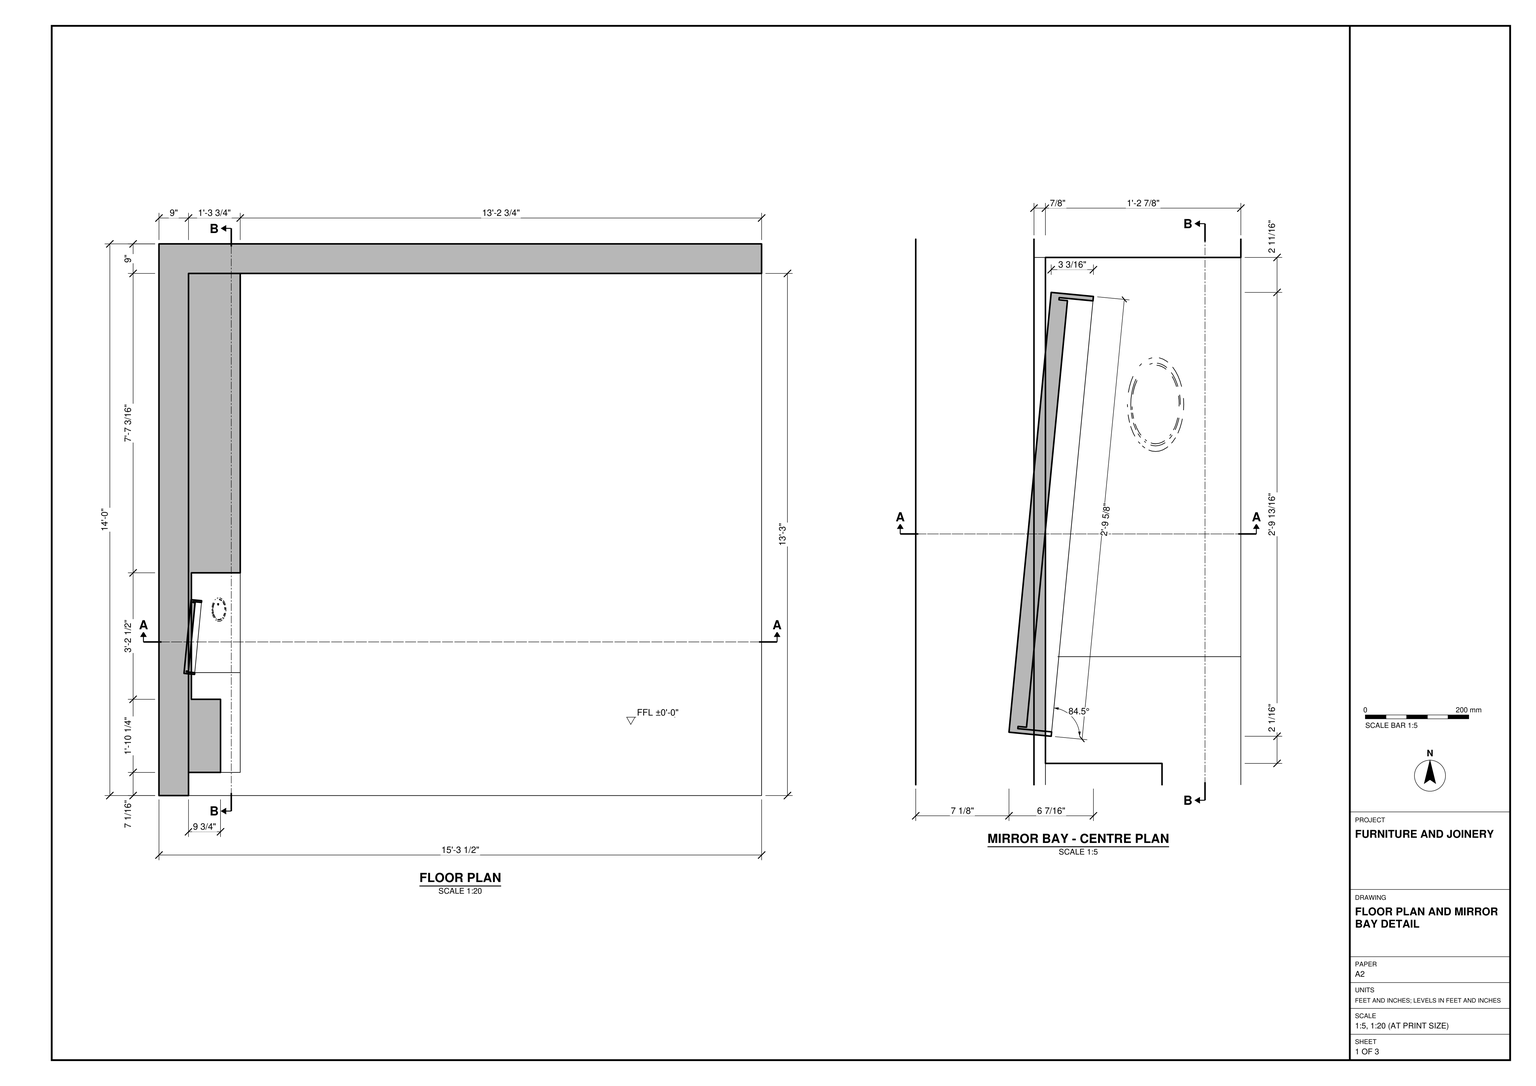
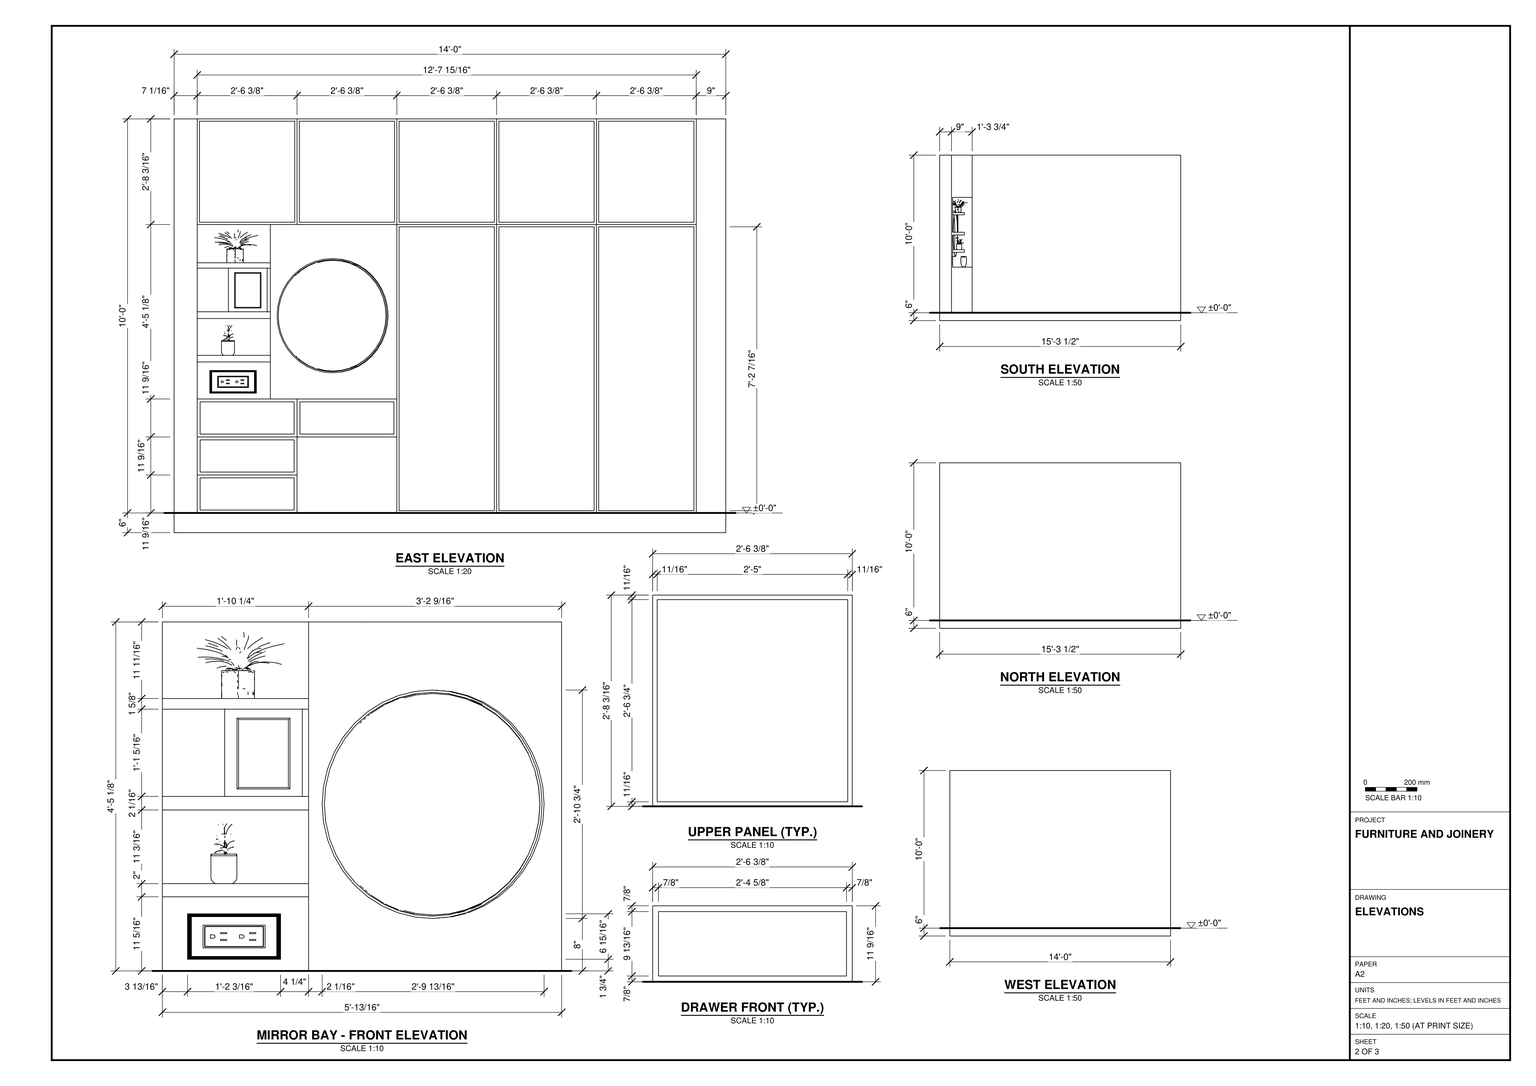
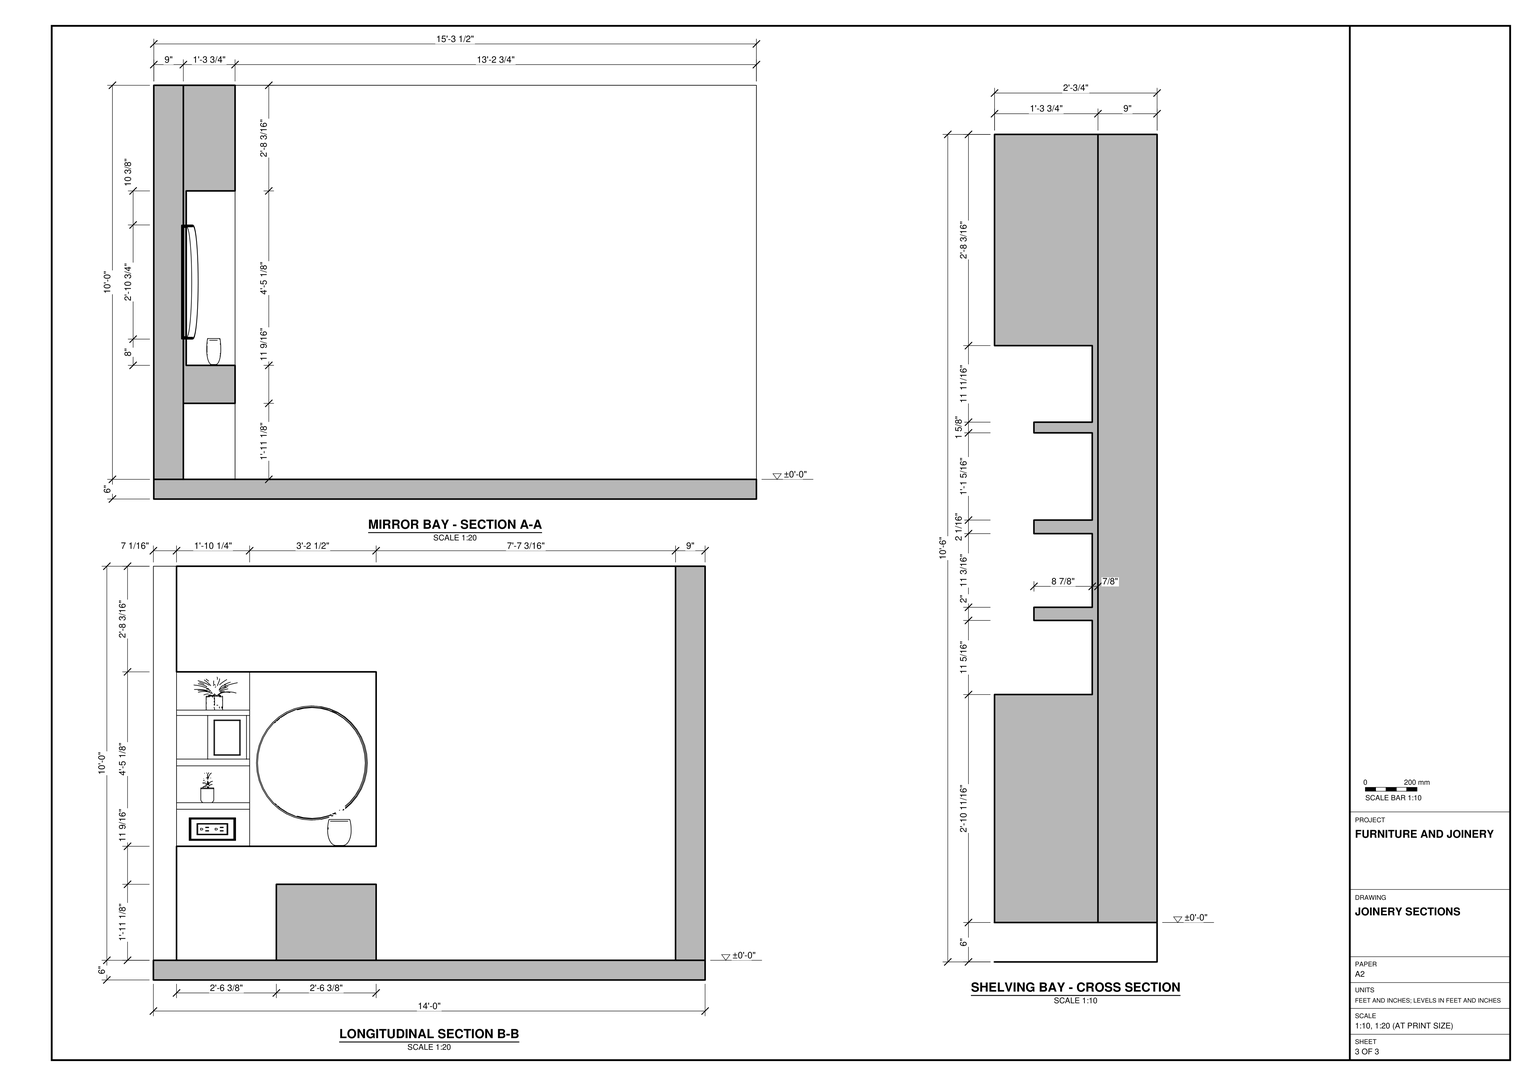
Use task_files/diagram_01.pdf to model the fitted storage wall and its room corner in SketchUp. Work in feet and inches. The overall model is 15'-3 1/2" along X, 14'-0" along Y and 10'-6" high. Set the finished floor at ±0'-0", with the 6" slab below it. Follow the floor plan for the two adjoining 9" walls, which rise 10'-0" above the finished floor.

Place the joinery against the wall shown in the east elevation. Run five equal upper panels across the top, with three tall fronts below them on the right. On the left, form the recessed bay with a narrow column of open shelves beside the round mirror. Use the enlarged plan to set the mirror at its slight angle to the wall. Below the recess, stack the drawer fronts on the left and extend the top drawer row beneath the mirror, leaving the space below open. Follow the panel details for the inset borders and the sections for the shelf and cabinet depths.

Include the shelf displays where shown; decor and loose items may be any suitable library components. Keep the walls, slab and each joinery piece in separate groups or components, and use components for repeated parts. Save one SketchUp model as output_files/fitted_storage_wall_with_a_recessed_mirror_bay.skp.

# SketchUp Ruby script. Lengths in inches.
U = 1.inch
M = Sketchup.active_model
def pt(a) = Geom::Point3d.new(a.map { |v| v * U })
def face(e, loops, mat)
  f = e.add_face(loops[0].map { |a| pt(a) })
  loops[1..].each { |l| e.add_face(l.map { |a| pt(a) }).erase! }
  f.material = f.back_material = mat if mat
  f
end
# faces: each face lists its corners as indices into pts; further lists are holes
def faces(e, pts, list, mat = nil) = list.each { |f| face(e, (f[0].is_a?(Array) ? f : [f]).map { |l| l.map { |i| pts[i] } }, mat) }
# xy, xz, yz: faces in a plane at the given z, y or x. An outline is a flat list of corners, or four numbers for a rectangle; further outlines are holes
def ring(l) = l.size == 4 ? [[l[0], l[1]], [l[2], l[1]], [l[2], l[3]], [l[0], l[3]]] : l.each_slice(2).to_a
def flat(e, list, mat, &to3) = list.each { |f| face(e, (f[0].is_a?(Array) ? f : [f]).map { |l| ring(l).map { |u, v| to3.(u, v) } }, mat) }
def xy(e, z, list, mat = nil) = flat(e, list, mat) { |x, y| [x, y, z] }
def xz(e, y, list, mat = nil) = flat(e, list, mat) { |x, z| [x, y, z] }
def yz(e, x, list, mat = nil) = flat(e, list, mat) { |y, z| [x, y, z] }
def lines(e, pts, list) = list.each { |a, b| e.add_line(pt(pts[a]), pt(pts[b])) }
# prism: a flat outline (further loops are holes) pulled along v
def prism(e, loops, v, mat = nil)
  f = face(e, loops, mat); d = Geom::Vector3d.new(v.map { |x| x * U })
  f.pushpull(f.normal.samedirection?(d) ? d.length : -d.length)
end
def box(e, o, s, mat = nil) = prism(e, [[o, [o[0] + s[0], o[1], o[2]], [o[0] + s[0], o[1] + s[1], o[2]], [o[0], o[1] + s[1], o[2]]]], [0, 0, s[2]], mat)
def at(x, y, z, deg = 0) = Geom::Transformation.translation(pt([x, y, z])) * Geom::Transformation.rotation(ORIGIN, Z_AXIS, deg.degrees)
def axes(o, x, y, z) = Geom::Transformation.new([*x, 0, *y, 0, *z, 0, *pt(o).to_a, 1])
def part(name) = M.definitions.add(name)
# library, detail: a bought-in or finely detailed component or shape, given as its bounding box
def library(name, o, s) = part(name).tap { |d| box(d.entities, o, s) }
def detail(e, o, s) = box(e.add_group.entities, o, s)
def put(e, d, t, mat = nil) = e.add_instance(d, t).tap { |i| i.material = mat if mat }
def group(e, t, mat = nil) = e.add_group.tap { |g| g.transformation = t; g.material = mat if mat }.entities
root = M.entities
M.materials.add("[0111_SlateGray]").color = [112, 128, 144]
M.materials.add("[0136_Charcoal]").color = [35, 35, 35]
M.materials.add("[Color M01]1").color = [226, 226, 226]
M.materials.add("[Color M09]3").color = [0, 0, 0]
c1 = library("Potted plant",[-1.15,-1.29,0],[7.65,7.78,5.89])
c2 = library("Small Plant for Nightstand",[-0.92,-1.74,0],[6.62,5.06,9.81])
c3 = part("Groupe\#1")
xy(c3.entities,0,[[0,0,24.58,0.41]])
xy(c3.entities,4.4,[[4.4,0.21,20.18,0.41]])
xy(c3.entities,28.07,[[4.4,0.21,20.18,0.41]])
xy(c3.entities,32.47,[[0,0,24.58,0.41]])
xz(c3.entities,0,[[[0,0,24.58,32.47],[3.9,3.9,20.68,28.57]]])
xz(c3.entities,0.41,[[[0,0,24.58,32.47],[4.4,4.4,20.18,28.07]]])
yz(c3.entities,0,[[0,0,0.41,32.47]])
yz(c3.entities,4.4,[[0.21,4.4,0.41,28.07]])
yz(c3.entities,20.18,[[0.21,4.4,0.41,28.07]])
yz(c3.entities,24.58,[[0,0,0.41,32.47]])
p = [[4.4,0.21,4.4],[4.4,0.21,28.07],[3.9,0,28.57],[3.9,0,3.9],[20.68,0,3.9],[20.18,0.21,4.4],
  [20.18,0.21,28.07],[20.68,0,28.57]]
faces(c3.entities,p,[[0,1,2,3],[3,4,5,0],[6,5,4,7],[1,6,7,2]])
c4 = part("Groupe\#3")
put(c4.entities,c3,axes([0.98,1.09,0.98],[0.7,0,0],[0,0.308,0],[0,0,0.7]))
c5 = part("Voile")
put(c5.entities,c4,axes([0,-0.3125,0],[0.9604,0,0],[0,0.9604,0],[0,0,0.9604]))
c6 = library("House Plant - small",[0,0,0],[36.52,33.08,30.88])
c7 = part("Picture frame")
g1 = group(c7.entities,at(0,0.03,3.15))
g2 = group(g1,at(0.79,-0.2,-0.79),"[Color M01]1")
prism(g2,[[[3.15,0.2,-1.57],[0,0.2,-1.57],[0,0.2,0],[3.15,0.2,0]],[[0.08,0.2,-1.5],[1.61,0.2,-1.5],[3.07,0.2,-1.5],[3.07,0.2,-0.08],[1.61,0.2,-0.08],[0.08,0.2,-0.08]]],[0,-0.28,0])
g3 = group(g1,at(0,0,0),"[Color M01]1")
xy(g3,-3.15,[[0,-0.05,4.72,-0.03],[0,-0.03,4.72,0]])
xy(g3,-2.36,[[0.79,-0.2,3.9375,0]])
xy(g3,-0.79,[[0.79,-0.2,3.9375,0]])
xy(g3,0,[[0,-0.05,4.72,-0.03],[0,-0.03,4.72,0]])
xz(g3,-0.2,[[0.17,-2.98,0.2,-2.95,0.2,-0.2,0.17,-0.17],[0.17,-2.98,4.55,-2.98,4.53,-2.95,0.2,-2.95],[4.55,-2.98,4.55,-0.17,4.53,-0.2,4.53,-2.95],[[0.2,-2.95,4.53,-0.2],[0.79,-2.36,3.9375,-0.79]],[0.2,-0.2,4.53,-0.2,4.55,-0.17,0.17,-0.17]])
xz(g3,-0.19,[[0.12,-3.03,0.14,-3,0.14,-0.14,0.12,-0.12],[0.12,-3.03,4.6,-3.03,4.58,-3,0.14,-3],[4.6,-3.03,4.6,-0.12,4.58,-0.14,4.58,-3],[0.14,-0.14,4.58,-0.14,4.6,-0.12,0.12,-0.12]])
xz(g3,0,[[[0,-3.15,4.72,0],[0.79,-2.36,3.9375,-0.79]]])
yz(g3,0,[[-0.05,-3.15,-0.03,0],[-0.03,-3.15,0,0]])
yz(g3,0.79,[[-0.2,-2.36,0,-0.79]])
yz(g3,3.9375,[[-0.2,-2.36,0,-0.79]])
yz(g3,4.72,[[-0.05,-3.15,-0.03,0],[-0.03,-3.15,0,0]])
p = [[4.67,-0.14,-3.1],[4.65,-0.16,-3.08],[0.07,-0.16,-3.08],[0.05,-0.14,-3.1],[4.63,-0.17,-3.05],[0.1,-0.17,-3.05],
  [4.6,-0.19,-3.03],[0.12,-0.19,-3.03],[0.07,-0.16,-1.57],[0.07,-0.16,-0.07],[0.05,-0.14,-0.05],[0.05,-0.14,-1.57],
  [0.1,-0.17,-1.57],[0.1,-0.17,-0.1],[0.12,-0.19,-1.57],[0.12,-0.19,-0.12],[4.65,-0.16,-0.07],[4.63,-0.17,-0.1],
  [4.6,-0.19,-0.12],[4.67,-0.14,-0.05],[4.72,-0.05,-3.15],[4.71,-0.08,-3.14],[0.01,-0.08,-3.14],[0,-0.05,-3.15],
  [4.7,-0.1,-3.125],[0.02,-0.1,-3.125],[4.6875,-0.12,-3.11],[0.04,-0.12,-3.11],[0.02,-0.1,-1.57],[0.02,-0.1,-0.02],
  [0.01,-0.08,-0.01],[0.01,-0.08,-1.57],[0,-0.05,0],[0,-0.05,-1.57],[0.04,-0.12,-0.04],[0.04,-0.12,-1.57],
  [4.72,-0.05,0],[4.71,-0.08,-0.01],[4.7,-0.1,-0.02],[4.6875,-0.12,-0.04],[4.58,-0.19,-3],[4.55,-0.2,-2.98],
  [0.17,-0.2,-2.98],[0.14,-0.19,-3],[0.17,-0.2,-1.57],[0.17,-0.2,-0.17],[0.14,-0.19,-0.14],[0.14,-0.19,-1.57],
  [4.58,-0.19,-0.14],[4.55,-0.2,-0.17]]
faces(g3,p,[[0,1,2,3],[1,4,5,2],[4,6,7,5],[3,2,8,9,10,11],[2,5,12,13,9,8],[5,7,14,15,13,12],[16,17,4,1],[17,18,6,4],
  [19,16,1,0],[20,21,22,23],[21,24,25,22],[24,26,27,25],[26,0,3,27],[22,25,28,29,30,31],[23,22,31,30,32,33],[27,3,11,10,34,35],
  [25,27,35,34,29,28],[36,37,21,20],[37,38,24,21],[38,39,26,24],[39,19,0,26],[40,41,42,43],[43,42,44,45,46,47],[48,49,41,40],
  [46,45,49,48],[10,9,16,19],[9,13,17,16],[13,15,18,17],[34,10,19,39],[32,30,37,36],[30,29,38,37],[29,34,39,38]])
g4 = group(g1,at(0.87,0,-0.87),"[Color M09]3")
box(g4,[0,-0.2,-1.42],[2.99,0.2,1.42])
g5 = group(g1,at(0.89,-0.24,-0.89))
prism(g5,[[[0,-0.04,-1.38],[2.95,-0.04,-1.38],[2.95,-0.04,0],[0,-0.04,0]],[[1.75,-0.04,-0.57],[1.87,-0.04,-0.57],[1.9,-0.04,-0.57],[1.93,-0.04,-0.59],[1.95,-0.04,-0.61],[1.97,-0.04,-0.63],[1.98,-0.04,-0.66],[1.99,-0.04,-0.6875],[1.98,-0.04,-0.72],[1.97,-0.04,-0.75],[1.95,-0.04,-0.77],[1.93,-0.04,-0.79],[1.9,-0.04,-0.8],[1.87,-0.04,-0.81],[1.75,-0.04,-0.81]],[[0.42,-0.04,-0.8],[0.39,-0.04,-0.81],[0.28,-0.04,-0.81],[0.28,-0.04,-0.57],[0.39,-0.04,-0.57],[0.42,-0.04,-0.57],[0.45,-0.04,-0.59],[0.48,-0.04,-0.61],[0.5,-0.04,-0.63],[0.51,-0.04,-0.66],[0.51,-0.04,-0.6875],[0.51,-0.04,-0.72],[0.5,-0.04,-0.75],[0.48,-0.04,-0.77],[0.45,-0.04,-0.79]],[[0.79,-0.04,-0.41],[1.1,-0.04,-0.41],[1.1,-0.04,-0.49],[0.79,-0.04,-0.49]],[[0.79,-0.04,-0.89],[1.1,-0.04,-0.89],[1.1,-0.04,-0.96],[0.79,-0.04,-0.96]],[[2.26,-0.04,-0.41],[2.58,-0.04,-0.41],[2.58,-0.04,-0.49],[2.26,-0.04,-0.49]],[[2.26,-0.04,-0.89],[2.58,-0.04,-0.89],[2.58,-0.04,-0.96],[2.26,-0.04,-0.96]]],[0,0.04,0],"[Color M01]1")
c8 = library("Group\#3",[-2.78,0.01,0],[6.43,33.79,34.77])
xz(root,168,[[0,0,183.5,120]])
put(root,c1,axes([15.59,52.48,34.71],[1,0,0],[0,1.67,0],[0,0,2.31222]))
put(root,c2,at(12.58,15.57,47.99))
put(root,c5,axes([17.04,15.86,60.09],[0,0.71501,0],[-4.25,0,0],[0,0,0.65]))
put(root,c6,axes([8.14,12.32,76.18],[0.35719,0,0],[0,0.4005,0],[0,0,0.33033]))
put(root,c7,axes([9.625,10.88,36.48],[0,3,0],[-1.00094,0,0],[0,0,2.197]))
g6 = group(root,at(0,0,-6))
box(g6,[0,0,0],[183.5,168,6])
g7 = group(root,at(0,0,0))
xy(g7,120,[[0,0,9,0,9,159,183.5,159,183.5,168,0,168]])
xz(g7,0,[[0,0,9,120]])
xz(g7,159,[[9,0,183.5,120]])
yz(g7,0,[[0,0,168,120]])
yz(g7,9,[[0,0,159,120]])
yz(g7,183.5,[[159,0,168,120]])
p = [[183.5,159,0],[183.5,0,0]]
lines(g7,p,[[0,1]])
g8 = group(root,at(9,7.05,0))
xy(g8,0,[[0,0,15.75,30.39],[0,60.78,15.75,151.95]])
xy(g8,23.14,[[0,30.39,15.75,60.78]])
xy(g8,34.71,[[0.875,0,15.75,30.39],[0.875,30.39,15.75,60.78]],"[0111_SlateGray]")
xy(g8,45.99,[[0.875,0,9.75,22.26]])
xy(g8,47.99,[[0.875,0,9.75,22.26]])
xy(g8,59.21,[[0.875,0,9.75,22.26]])
xy(g8,61.28,[[0.875,0,9.75,22.26]])
xy(g8,74.56,[[0.875,0,9.75,22.26]])
xy(g8,76.18,[[0.875,0,9.75,22.26]])
xy(g8,87.84,[[0.875,0,15.75,30.39],[0.875,30.39,15.75,60.78]],"[0111_SlateGray]")
xy(g8,120,[[0,0,15.75,151.95]])
xz(g8,0,[[0,0,15.75,0,15.75,34.71,0.875,34.71,0.875,59.21,9.75,59.21,9.75,61.28,0.875,61.28,0.875,87.84,15.75,87.84,15.75,120,0,120],[0.875,45.99,9.75,47.99],[0.875,74.56,9.75,76.18]],"[0111_SlateGray]")
xz(g8,22.26,[[0.875,45.99,9.75,47.99],[0.875,59.21,9.75,61.28],[0.875,74.56,9.75,76.18]])
xz(g8,30.39,[[0,0,15.75,11.57],[0,11.57,15.75,23.14]])
xz(g8,60.78,[[0,0,15.75,23.14],[0.875,34.71,15.75,87.84]],"[0111_SlateGray]")
xz(g8,151.95,[[0,0,15.75,120]])
yz(g8,0,[[0,0,0,120,151.95,120,151.95,0,60.78,0,60.78,23.14,30.39,23.14,30.39,0]])
yz(g8,0,[[-7.05,0,0,120],[30.39,0,60.78,23.14]],"[0111_SlateGray]")
yz(g8,0.875,[[0,34.71,22.26,45.99],[22.26,34.71,60.78,87.84],[0,47.99,22.26,59.21],[0,61.28,22.26,74.56],[0,76.18,22.26,87.84]])
yz(g8,9.75,[[0,45.99,22.26,47.99],[0,59.21,22.26,61.28],[0,74.56,22.26,76.18]],"[0136_Charcoal]")
yz(g8,15.75,[[[0,0,30.39,11.57],[0.88,0.88,29.51,10.6875]],[61.47,0.69,90.48,87.15],[91.86,0.69,120.87,87.15],[122.25,0.69,151.26,87.15],[0.88,0.88,29.51,10.6875],
  [[0,11.57,30.39,23.14],[0.88,12.45,29.51,22.26]],[0.88,12.45,29.51,22.26],[[0,23.14,30.39,34.71],[0.88,24.02,29.51,33.83]],[[30.39,23.14,60.78,34.71],[31.27,24.02,59.9,33.83]],[0.88,24.02,29.51,33.83],
  [31.27,24.02,59.9,33.83],[0.69,88.53,29.7,119.31],[31.08,88.53,60.09,119.31],[61.47,88.53,90.48,119.31],[91.86,88.53,120.87,119.31],
  [122.25,88.53,151.26,119.31]],"[0111_SlateGray]")
yz(g8,15.75,[[[60.78,0,91.17,87.84],[61.47,0.69,90.48,87.15]],[[91.17,0,121.5625,87.84],[91.86,0.69,120.87,87.15]],[[121.5625,0,151.95,87.84],[122.25,0.69,151.26,87.15]],[[0,87.84,30.39,120],[0.69,88.53,29.7,119.31]],[[30.39,87.84,60.78,120],[31.08,88.53,60.09,119.31]],
  [[60.78,87.84,91.17,120],[61.47,88.53,90.48,119.31]],[[91.17,87.84,121.5625,120],[91.86,88.53,120.87,119.31]],[[121.5625,87.84,151.95,120],[122.25,88.53,151.26,119.31]]],"[0136_Charcoal]")
put(root,c8,at(9.875,31.37,42.7))
